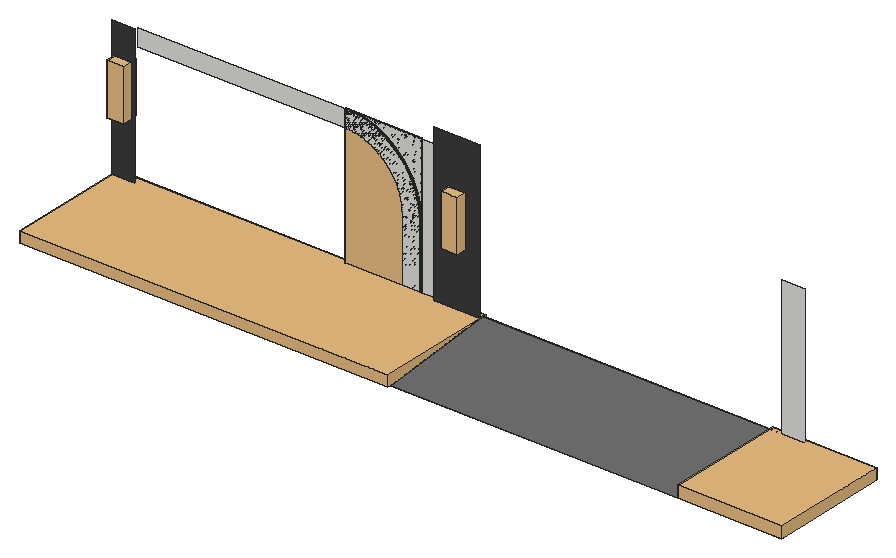
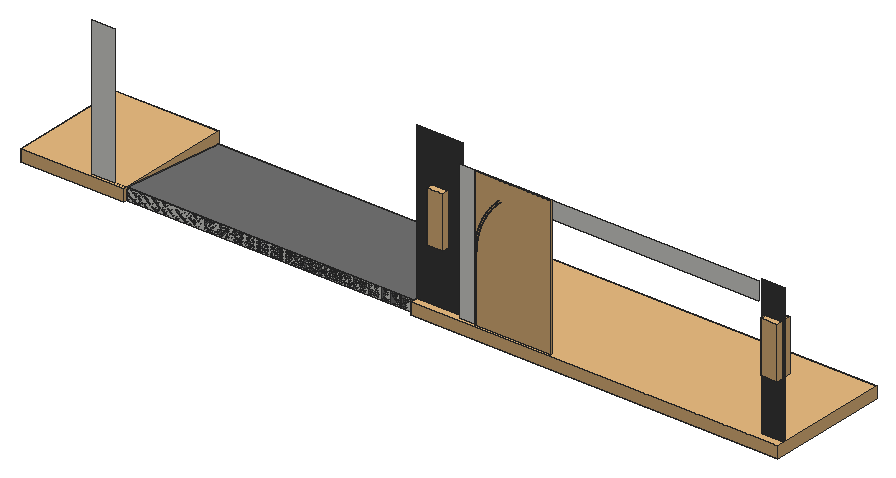
# SketchUp Ruby script. Lengths in inches.
U = 1.inch
M = Sketchup.active_model
def pt(a) = Geom::Point3d.new(a.map { |v| v * U })
def face(e, loops, mat)
  f = e.add_face(loops[0].map { |a| pt(a) })
  loops[1..].each { |l| e.add_face(l.map { |a| pt(a) }).erase! }
  f.material = f.back_material = mat if mat
  f
end
# faces: each face lists its corners as indices into pts; further lists are holes
def faces(e, pts, list, mat = nil) = list.each { |f| face(e, (f[0].is_a?(Array) ? f : [f]).map { |l| l.map { |i| pts[i] } }, mat) }
# xy, xz, yz: faces in a plane at the given z, y or x. An outline is a flat list of corners, or four numbers for a rectangle; further outlines are holes
def ring(l) = l.size == 4 ? [[l[0], l[1]], [l[2], l[1]], [l[2], l[3]], [l[0], l[3]]] : l.each_slice(2).to_a
def flat(e, list, mat, &to3) = list.each { |f| face(e, (f[0].is_a?(Array) ? f : [f]).map { |l| ring(l).map { |u, v| to3.(u, v) } }, mat) }
def xy(e, z, list, mat = nil) = flat(e, list, mat) { |x, y| [x, y, z] }
def xz(e, y, list, mat = nil) = flat(e, list, mat) { |x, z| [x, y, z] }
def yz(e, x, list, mat = nil) = flat(e, list, mat) { |y, z| [x, y, z] }
def lines(e, pts, list) = list.each { |a, b| e.add_line(pt(pts[a]), pt(pts[b])) }
# prism: a flat outline (further loops are holes) pulled along v
def prism(e, loops, v, mat = nil)
  f = face(e, loops, mat); d = Geom::Vector3d.new(v.map { |x| x * U })
  f.pushpull(f.normal.samedirection?(d) ? d.length : -d.length)
end
def box(e, o, s, mat = nil) = prism(e, [[o, [o[0] + s[0], o[1], o[2]], [o[0] + s[0], o[1] + s[1], o[2]], [o[0], o[1] + s[1], o[2]]]], [0, 0, s[2]], mat)
def at(x, y, z, deg = 0) = Geom::Transformation.translation(pt([x, y, z])) * Geom::Transformation.rotation(ORIGIN, Z_AXIS, deg.degrees)
def axes(o, x, y, z) = Geom::Transformation.new([*x, 0, *y, 0, *z, 0, *pt(o).to_a, 1])
def part(name) = M.definitions.add(name)
# library, detail: a bought-in or finely detailed component or shape, given as its bounding box
def library(name, o, s) = part(name).tap { |d| box(d.entities, o, s) }
def detail(e, o, s) = box(e.add_group.entities, o, s)
def put(e, d, t, mat = nil) = e.add_instance(d, t).tap { |i| i.material = mat if mat }
def group(e, t, mat = nil) = e.add_group.tap { |g| g.transformation = t; g.material = mat if mat }.entities
root = M.entities
M.materials.add("Outer light").color = [250, 223, 139]
M.materials.add("[Granite Dark Gray]").color = [61, 60, 60]
M.materials.add("[Granite Tile]").color = [112, 112, 112]
c1 = library("Group\#30",[-12,0,0],[192,64,6])
c2 = library("Group\#31",[0,-48,0],[54,62,6])
c3 = library("WALL LIGHT 61",[-1.86,-2.6875,-10.98],[8.43,8.43,26.69])
c4 = library("Group\#28",[0,-0.5,0],[40,0.5,78])
xz(root,58,[[0,-12,12,66],[168,-12,192,75]],"[Granite Dark Gray]")
xz(root,60,[[150,-12,159,-12,159,27.51,158.99,28.02,158.95,29.04,158.92,29.55,158.84,30.57,158.79,31.08,158.73,31.58,158.67,32.09,158.6,32.6,158.52,33.1,158.4375,33.6,158.35,34.11,158.15,35.11,158.04,35.61,157.92,36.1,157.8,36.6,157.67,37.09,157.54,37.59,157.39,38.08,157.25,38.57,157.09,39.05,156.93,39.54,156.59,40.5,156.41,40.98,156.03,41.92,155.83,42.4,155.63,42.86,155.42,43.33,154.98,44.25,154.75,44.71,154.03,46.06,153.77,46.5,153.52,46.94,153.25,47.38,152.98,47.8125,152.71,48.24,152.43,48.67,151.85,49.51,151.25,50.33,150.94,50.74,150.63,51.14,150.31,51.54,149.98,51.9375,149.66,52.33,149.32,52.71,148.98,53.1,148.64,53.47,148.29,53.85,147.9375,54.21,147.58,54.58,147.21,54.9375,146.85,55.29,146.47,55.64,146.1,55.98,145.71,56.32,145.33,56.66,144.9375,56.98,144.54,57.31,144.14,57.63,143.74,57.94,143.33,58.25,142.51,58.85,141.67,59.43,141.24,59.71,140.8125,59.98,140.38,60.25,139.94,60.52,139.5,60.77,139.06,61.03,137.71,61.75,137.25,61.98,136.33,62.42,135.86,62.63,135.4,62.83,134.92,63.03,133.98,63.41,133.5,63.59,132.54,63.93,132.05,64.09,131.57,64.25,131.08,64.39,130.59,64.54,130.09,64.67,129.6,64.8,129.1,64.92,128.61,65.04,128.11,65.15,127.11,65.35,126.6,65.4375,126.1,65.52,125.6,65.6,125.09,65.67,124.58,65.73,124.08,65.79,123.57,65.84,122.55,65.92,122.04,65.95,121.02,65.99,120.51,66,12,66,12,57,120.39,57,120.79,56.99,121.18,56.98,121.57,56.96,121.96,56.9375,122.35,56.91,122.75,56.875,123.14,56.84,123.92,56.74,124.3,56.69,125.08,56.57,125.47,56.5,125.85,56.42,126.24,56.34,126.62,56.26,127.38,56.08,127.76,55.98,128.14,55.875,128.52,55.76,128.9,55.65,129.64,55.41,130.38,55.15,130.75,55.01,131.12,54.86,131.48,54.72,131.84,54.5625,132.2,54.41,132.56,54.24,132.92,54.08,133.27,53.91,133.97,53.55,134.31,53.36,134.66,53.17,135,52.98,135.34,52.78,135.67,52.58,136.01,52.37,136.34,52.16,136.67,51.94,136.99,51.72,137.3125,51.5,137.63,51.27,137.95,51.04,138.57,50.56,138.88,50.3125,139.18,50.07,139.48,49.8125,139.78,49.56,140.07,49.29,140.36,49.03,140.65,48.76,140.93,48.49,141.49,47.93,141.76,47.65,142.03,47.36,142.29,47.07,142.56,46.78,142.8125,46.48,143.07,46.18,143.3125,45.88,143.56,45.57,144.04,44.95,144.27,44.63,144.5,44.3125,144.72,43.99,144.94,43.67,145.16,43.34,145.37,43.01,145.58,42.67,145.78,42.34,145.98,42,146.17,41.66,146.36,41.31,146.55,40.97,146.91,40.27,147.08,39.92,147.24,39.56,147.41,39.2,147.5625,38.84,147.72,38.48,147.86,38.12,148.01,37.75,148.15,37.38,148.41,36.64,148.65,35.9,148.76,35.52,148.875,35.14,148.98,34.76,149.08,34.38,149.26,33.62,149.34,33.24,149.42,32.85,149.5,32.47,149.57,32.08,149.69,31.3,149.74,30.92,149.84,30.14,149.875,29.75,149.91,29.35,149.9375,28.96,149.96,28.57,149.98,28.18,149.99,27.79,150,27.39],[160,-12,168,-12,168,66,128.89,66,129.34,65.89,129.85,65.77,130.35,65.64,130.86,65.5,131.86,65.2,132.86,64.88,133.35,64.71,133.84,64.53,135.31,63.96,136.75,63.33,137.22,63.1,137.69,62.875,138.16,62.64,138.625,62.4,139.09,62.15,139.54,61.9,140,61.64,140.9,61.11,141.34,60.83,141.79,60.55,142.22,60.26,142.66,59.97,143.09,59.67,143.93,59.05,144.35,58.73,145.17,58.09,145.58,57.75,145.98,57.42,146.375,57.07,146.77,56.73,147.91,55.65,148.65,54.91,149.73,53.77,150.07,53.375,150.42,52.98,150.75,52.58,151.09,52.17,151.73,51.35,152.05,50.93,152.67,50.09,152.97,49.66,153.26,49.22,153.55,48.79,153.83,48.34,154.11,47.9,154.64,47,154.9,46.54,155.15,46.09,155.4,45.625,155.64,45.16,155.875,44.69,156.1,44.22,156.33,43.75,156.96,42.31,157.53,40.84,157.71,40.35,157.88,39.86,158.2,38.86,158.5,37.86,158.64,37.35,158.77,36.85,159.01,35.83,159.125,35.32,159.23,34.8,159.33,34.29,159.42,33.77,159.51,33.26,159.59,32.74,159.66,32.22,159.78,31.18,159.83,30.66,159.875,30.14,159.91,29.62,159.95,29.09,159.99,28.05,160,27.52],[192,-12,360,-12,360,66,348,66,348,-6,192,-6]])
yz(root,159,[[60,-12,60.5,27],[60,27,60.5,27.51]])
yz(root,160,[[60,-12,60.5,27],[60,27,60.5,27.52]])
p = [[158.99,60,28.02],[159,60,27.51],[159,60.5,27.51],[158.99,60.5,28.02],[160,60,27.52],[159.99,60,28.05],
  [159.99,60.5,28.05],[160,60.5,27.52],[158.97,60,28.53],[158.97,60.5,28.53],[159.97,60,28.57],[159.97,60.5,28.57],
  [158.95,60,29.04],[158.95,60.5,29.04],[159.95,60,29.09],[159.95,60.5,29.09],[158.92,60,29.55],[158.92,60.5,29.55],
  [159.91,60,29.62],[159.91,60.5,29.62],[158.88,60,30.06],[158.88,60.5,30.06],[159.875,60,30.14],[159.875,60.5,30.14],
  [158.84,60,30.57],[158.84,60.5,30.57],[159.83,60,30.66],[159.83,60.5,30.66],[158.79,60,31.08],[158.79,60.5,31.08],
  [159.78,60,31.18],[159.78,60.5,31.18],[158.73,60,31.58],[158.73,60.5,31.58],[159.72,60,31.7],[159.72,60.5,31.7],
  [158.67,60,32.09],[158.67,60.5,32.09],[159.66,60,32.22],[159.66,60.5,32.22],[158.6,60,32.6],[158.6,60.5,32.6],
  [159.59,60,32.74],[159.59,60.5,32.74],[158.52,60,33.1],[158.52,60.5,33.1],[159.51,60,33.26],[159.51,60.5,33.26],
  [158.4375,60,33.6],[158.4375,60.5,33.6],[159.42,60,33.77],[159.42,60.5,33.77],[158.35,60,34.11],[158.35,60.5,34.11],
  [159.33,60,34.29],[159.33,60.5,34.29],[158.25,60,34.61],[158.25,60.5,34.61],[159.23,60,34.8],[159.23,60.5,34.8],
  [158.15,60,35.11],[158.15,60.5,35.11],[159.125,60,35.32],[159.125,60.5,35.32],[158.04,60,35.61],[158.04,60.5,35.61],
  [159.01,60,35.83],[159.01,60.5,35.83],[157.92,60,36.1],[157.92,60.5,36.1],[158.89,60,36.34],[158.89,60.5,36.34],
  [157.8,60,36.6],[157.8,60.5,36.6],[158.77,60,36.85],[158.77,60.5,36.85],[157.67,60,37.09],[157.67,60.5,37.09],
  [158.64,60,37.35],[158.64,60.5,37.35],[157.54,60,37.59],[157.54,60.5,37.59],[158.5,60,37.86],[158.5,60.5,37.86],
  [157.39,60,38.08],[157.39,60.5,38.08],[158.35,60,38.36],[158.35,60.5,38.36],[157.25,60,38.57],[157.25,60.5,38.57],
  [158.2,60,38.86],[158.2,60.5,38.86],[157.09,60,39.05],[157.09,60.5,39.05],[158.04,60,39.36],[158.04,60.5,39.36],
  [156.93,60,39.54],[156.93,60.5,39.54],[157.88,60,39.86],[157.88,60.5,39.86],[156.76,60,40.02],[156.76,60.5,40.02],
  [157.71,60,40.35],[157.71,60.5,40.35],[156.59,60,40.5],[156.59,60.5,40.5],[157.53,60,40.84],[157.53,60.5,40.84],
  [156.41,60,40.98],[156.41,60.5,40.98],[157.34,60,41.33],[157.34,60.5,41.33],[156.22,60,41.45],[156.22,60.5,41.45],
  [157.15,60,41.82],[157.15,60.5,41.82],[156.03,60,41.92],[156.03,60.5,41.92],[156.96,60,42.31],[156.96,60.5,42.31],
  [155.83,60,42.4],[155.83,60.5,42.4],[156.75,60,42.79],[156.75,60.5,42.79],[155.63,60,42.86],[155.63,60.5,42.86],
  [156.54,60,43.27],[156.54,60.5,43.27],[155.42,60,43.33],[155.42,60.5,43.33],[155.2,60,43.79],[155.2,60.5,43.79],
  [156.33,60,43.75],[156.33,60.5,43.75],[156.1,60,44.22],[156.1,60.5,44.22],[154.98,60,44.25],[154.98,60.5,44.25],
  [154.75,60,44.71],[154.75,60.5,44.71],[155.875,60,44.69],[155.875,60.5,44.69],[154.51,60,45.16],[154.51,60.5,45.16],
  [155.64,60,45.16],[155.64,60.5,45.16],[154.27,60,45.61],[154.27,60.5,45.61],[155.4,60,45.625],[155.4,60.5,45.625],
  [154.03,60,46.06],[154.03,60.5,46.06],[155.15,60,46.09],[155.15,60.5,46.09],[153.77,60,46.5],[153.77,60.5,46.5],
  [154.9,60,46.54],[154.9,60.5,46.54],[153.52,60,46.94],[153.52,60.5,46.94],[154.64,60,47],[154.64,60.5,47],
  [153.25,60,47.38],[153.25,60.5,47.38],[154.375,60,47.45],[154.375,60.5,47.45],[152.98,60,47.8125],[152.98,60.5,47.8125],
  [154.11,60,47.9],[154.11,60.5,47.9],[152.71,60,48.24],[152.71,60.5,48.24],[153.83,60,48.34],[153.83,60.5,48.34],
  [152.43,60,48.67],[152.43,60.5,48.67],[153.55,60,48.79],[153.55,60.5,48.79],[152.14,60,49.09],[152.14,60.5,49.09],
  [153.26,60,49.22],[153.26,60.5,49.22],[151.85,60,49.51],[151.85,60.5,49.51],[152.97,60,49.66],[152.97,60.5,49.66],
  [151.55,60,49.92],[151.55,60.5,49.92],[152.67,60,50.09],[152.67,60.5,50.09],[151.25,60,50.33],[151.25,60.5,50.33],
  [152.36,60,50.51],[152.36,60.5,50.51],[150.94,60,50.74],[150.94,60.5,50.74],[152.05,60,50.93],[152.05,60.5,50.93],
  [150.63,60,51.14],[150.63,60.5,51.14],[151.73,60,51.35],[151.73,60.5,51.35],[150.31,60,51.54],[150.31,60.5,51.54],
  [151.41,60,51.76],[151.41,60.5,51.76],[149.98,60,51.9375],[149.98,60.5,51.9375],[151.09,60,52.17],[151.09,60.5,52.17],
  [149.66,60,52.33],[149.66,60.5,52.33],[150.75,60,52.58],[150.75,60.5,52.58],[149.32,60,52.71],[149.32,60.5,52.71],
  [150.42,60,52.98],[150.42,60.5,52.98],[148.98,60,53.1],[148.98,60.5,53.1],[150.07,60,53.375],[150.07,60.5,53.375],
  [148.64,60,53.47],[148.64,60.5,53.47],[149.73,60,53.77],[149.73,60.5,53.77],[148.29,60,53.85],[148.29,60.5,53.85],
  [147.9375,60,54.21],[147.9375,60.5,54.21],[149.37,60,54.15],[149.37,60.5,54.15],[147.58,60,54.58],[147.58,60.5,54.58],
  [149.01,60,54.53],[149.01,60.5,54.53],[148.65,60,54.91],[148.65,60.5,54.91],[147.21,60,54.9375],[147.21,60.5,54.9375],
  [146.85,60,55.29],[146.85,60.5,55.29],[148.28,60,55.28],[148.28,60.5,55.28],[146.47,60,55.64],[146.47,60.5,55.64],
  [147.91,60,55.65],[147.91,60.5,55.65],[146.1,60,55.98],[146.1,60.5,55.98],[147.53,60,56.01],[147.53,60.5,56.01],
  [145.71,60,56.32],[145.71,60.5,56.32],[147.15,60,56.37],[147.15,60.5,56.37],[145.33,60,56.66],[145.33,60.5,56.66],
  [146.77,60,56.73],[146.77,60.5,56.73],[144.9375,60,56.98],[144.9375,60.5,56.98],[146.375,60,57.07],[146.375,60.5,57.07],
  [144.54,60,57.31],[144.54,60.5,57.31],[145.98,60,57.42],[145.98,60.5,57.42],[144.14,60,57.63],[144.14,60.5,57.63],
  [145.58,60,57.75],[145.58,60.5,57.75],[143.74,60,57.94],[143.74,60.5,57.94],[145.17,60,58.09],[145.17,60.5,58.09],
  [143.33,60,58.25],[143.33,60.5,58.25],[144.76,60,58.41],[144.76,60.5,58.41],[142.92,60,58.55],[142.92,60.5,58.55],
  [144.35,60,58.73],[144.35,60.5,58.73],[142.51,60,58.85],[142.51,60.5,58.85],[143.93,60,59.05],[143.93,60.5,59.05],
  [142.09,60,59.14],[142.09,60.5,59.14],[141.67,60,59.43],[141.67,60.5,59.43],[143.51,60,59.36],[143.51,60.5,59.36],
  [141.24,60,59.71],[141.24,60.5,59.71],[143.09,60,59.67],[143.09,60.5,59.67],[140.8125,60,59.98],[140.8125,60.5,59.98],
  [142.66,60,59.97],[142.66,60.5,59.97],[140.38,60,60.25],[140.38,60.5,60.25],[142.22,60,60.26],[142.22,60.5,60.26],
  [139.94,60,60.52],[139.94,60.5,60.52],[141.79,60,60.55],[141.79,60.5,60.55],[139.5,60,60.77],[139.5,60.5,60.77],
  [141.34,60,60.83],[141.34,60.5,60.83],[139.06,60,61.03],[139.06,60.5,61.03],[140.9,60,61.11],[140.9,60.5,61.11],
  [138.61,60,61.27],[138.61,60.5,61.27],[140.45,60,61.375],[140.45,60.5,61.375],[138.16,60,61.51],[138.16,60.5,61.51],
  [140,60,61.64],[140,60.5,61.64],[137.71,60,61.75],[137.71,60.5,61.75],[139.54,60,61.9],[139.54,60.5,61.9],
  [137.25,60,61.98],[137.25,60.5,61.98],[139.09,60,62.15],[139.09,60.5,62.15],[136.79,60,62.2],[136.79,60.5,62.2],
  [136.33,60,62.42],[136.33,60.5,62.42],[138.625,60,62.4],[138.625,60.5,62.4],[135.86,60,62.63],[135.86,60.5,62.63],
  [138.16,60,62.64],[138.16,60.5,62.64],[135.4,60,62.83],[135.4,60.5,62.83],[137.69,60,62.875],[137.69,60.5,62.875],
  [134.92,60,63.03],[134.92,60.5,63.03],[137.22,60,63.1],[137.22,60.5,63.1],[134.45,60,63.22],[134.45,60.5,63.22],
  [136.75,60,63.33],[136.75,60.5,63.33],[133.98,60,63.41],[133.98,60.5,63.41],[136.27,60,63.54],[136.27,60.5,63.54],
  [133.5,60,63.59],[133.5,60.5,63.59],[135.79,60,63.75],[135.79,60.5,63.75],[133.02,60,63.76],[133.02,60.5,63.76],
  [135.31,60,63.96],[135.31,60.5,63.96],[192,48,-12],[342,48,-12]]
faces(root,p,[[0,1,2,3],[4,5,6,7],[8,0,3,9],[5,10,11,6],[12,8,9,13],[10,14,15,11],[16,12,13,17],[14,18,19,15],
  [20,16,17,21],[18,22,23,19],[24,20,21,25],[22,26,27,23],[28,24,25,29],[26,30,31,27],[32,28,29,33],[30,34,35,31],
  [36,32,33,37],[34,38,39,35],[40,36,37,41],[38,42,43,39],[44,40,41,45],[42,46,47,43],[48,44,45,49],[46,50,51,47],
  [52,48,49,53],[50,54,55,51],[56,52,53,57],[54,58,59,55],[60,56,57,61],[58,62,63,59],[64,60,61,65],[62,66,67,63],
  [68,64,65,69],[66,70,71,67],[72,68,69,73],[70,74,75,71],[76,72,73,77],[74,78,79,75],[80,76,77,81],[78,82,83,79],
  [84,80,81,85],[82,86,87,83],[88,84,85,89],[86,90,91,87],[92,88,89,93],[90,94,95,91],[96,92,93,97],[94,98,99,95],
  [100,96,97,101],[98,102,103,99],[104,100,101,105],[102,106,107,103],[108,104,105,109],[106,110,111,107],[112,108,109,113],[110,114,115,111],
  [116,112,113,117],[114,118,119,115],[120,116,117,121],[118,122,123,119],[124,120,121,125],[122,126,127,123],[128,124,125,129],[130,128,129,131],
  [126,132,133,127],[132,134,135,133],[136,130,131,137],[138,136,137,139],[134,140,141,135],[142,138,139,143],[140,144,145,141],[146,142,143,147],
  [144,148,149,145],[150,146,147,151],[148,152,153,149],[154,150,151,155],[152,156,157,153],[158,154,155,159],[156,160,161,157],[162,158,159,163],
  [160,164,165,161],[166,162,163,167],[164,168,169,165],[170,166,167,171],[168,172,173,169],[174,170,171,175],[172,176,177,173],[178,174,175,179],
  [176,180,181,177],[182,178,179,183],[180,184,185,181],[186,182,183,187],[184,188,189,185],[190,186,187,191],[188,192,193,189],[194,190,191,195],
  [192,196,197,193],[198,194,195,199],[196,200,201,197],[202,198,199,203],[200,204,205,201],[206,202,203,207],[204,208,209,205],[210,206,207,211],
  [208,212,213,209],[214,210,211,215],[212,216,217,213],[218,214,215,219],[216,220,221,217],[222,218,219,223],[220,224,225,221],[226,222,223,227],
  [228,226,227,229],[224,230,231,225],[232,228,229,233],[230,234,235,231],[234,236,237,235],[238,232,233,239],[240,238,239,241],[236,242,243,237],
  [244,240,241,245],[242,246,247,243],[248,244,245,249],[246,250,251,247],[252,248,249,253],[250,254,255,251],[256,252,253,257],[254,258,259,255],
  [260,256,257,261],[258,262,263,259],[264,260,261,265],[262,266,267,263],[268,264,265,269],[266,270,271,267],[272,268,269,273],[270,274,275,271],
  [276,272,273,277],[274,278,279,275],[280,276,277,281],[278,282,283,279],[284,280,281,285],[282,286,287,283],[288,284,285,289],[290,288,289,291],
  [286,292,293,287],[294,290,291,295],[292,296,297,293],[298,294,295,299],[296,300,301,297],[302,298,299,303],[300,304,305,301],[306,302,303,307],
  [304,308,309,305],[310,306,307,311],[308,312,313,309],[314,310,311,315],[312,316,317,313],[318,314,315,319],[316,320,321,317],[322,318,319,323],
  [320,324,325,321],[326,322,323,327],[324,328,329,325],[330,326,327,331],[328,332,333,329],[334,330,331,335],[336,334,335,337],[332,338,339,333],
  [340,336,337,341],[338,342,343,339],[344,340,341,345],[342,346,347,343],[348,344,345,349],[346,350,351,347],[352,348,349,353],[350,354,355,351],
  [356,352,353,357],[354,358,359,355],[360,356,357,361],[358,362,363,359],[364,360,361,365],[362,366,367,363]])
lines(root,p,[[368,369]])
put(root,c1,at(12,-2,-12),"[Granite Tile]")
g1 = group(root,at(192,60,-12),"[Granite Tile]")
prism(g1,[[[150,0,0],[150,0,6],[150,-60,0]]],[-150,0,0])
put(root,c2,at(342,48,-12),"[Granite Tile]")
put(root,c3,at(177.65,55.58,34.28))
put(root,c3,at(3.34,55.58,34.28))
put(root,c4,at(120,60.5,-12),"Outer light")
